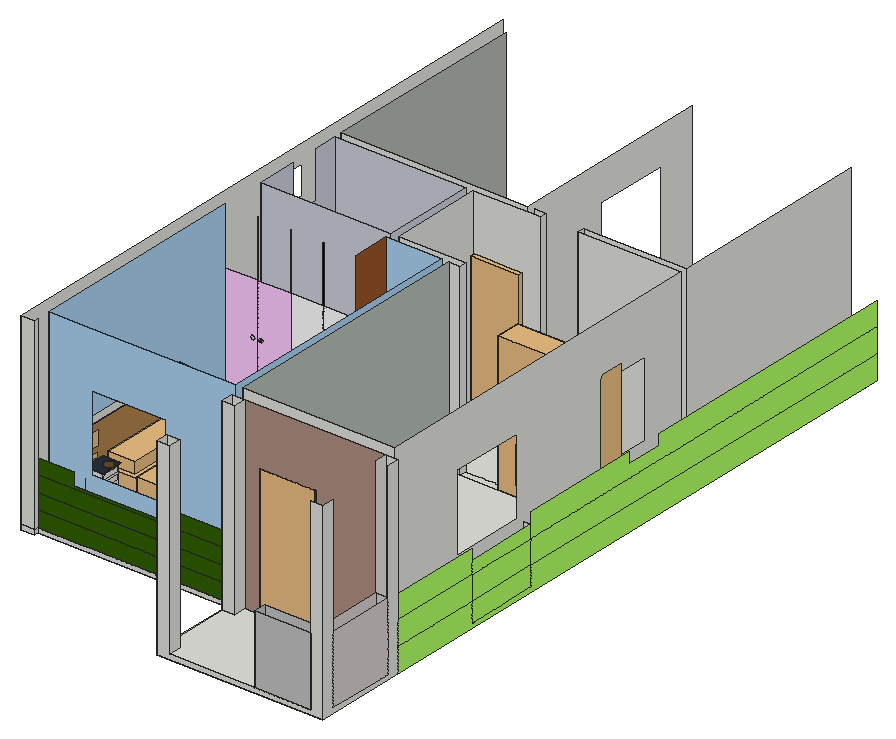
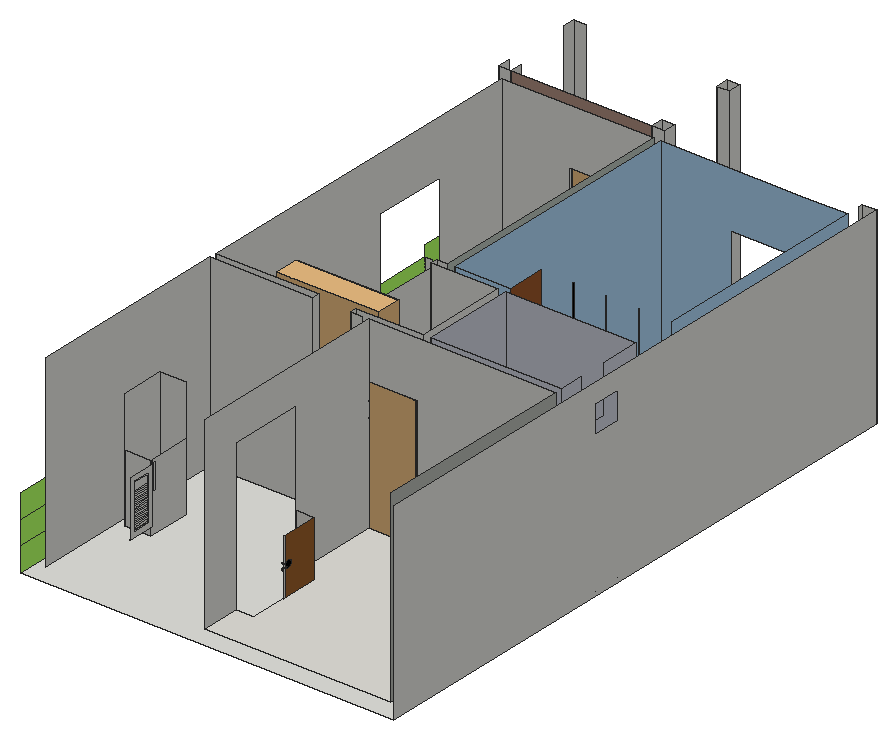
# SketchUp Ruby script. Lengths in inches.
U = 1.inch
M = Sketchup.active_model
def pt(a) = Geom::Point3d.new(a.map { |v| v * U })
def face(e, loops, mat)
  f = e.add_face(loops[0].map { |a| pt(a) })
  loops[1..].each { |l| e.add_face(l.map { |a| pt(a) }).erase! }
  f.material = f.back_material = mat if mat
  f
end
# faces: each face lists its corners as indices into pts; further lists are holes
def faces(e, pts, list, mat = nil) = list.each { |f| face(e, (f[0].is_a?(Array) ? f : [f]).map { |l| l.map { |i| pts[i] } }, mat) }
# xy, xz, yz: faces in a plane at the given z, y or x. An outline is a flat list of corners, or four numbers for a rectangle; further outlines are holes
def ring(l) = l.size == 4 ? [[l[0], l[1]], [l[2], l[1]], [l[2], l[3]], [l[0], l[3]]] : l.each_slice(2).to_a
def flat(e, list, mat, &to3) = list.each { |f| face(e, (f[0].is_a?(Array) ? f : [f]).map { |l| ring(l).map { |u, v| to3.(u, v) } }, mat) }
def xy(e, z, list, mat = nil) = flat(e, list, mat) { |x, y| [x, y, z] }
def xz(e, y, list, mat = nil) = flat(e, list, mat) { |x, z| [x, y, z] }
def yz(e, x, list, mat = nil) = flat(e, list, mat) { |y, z| [x, y, z] }
def lines(e, pts, list) = list.each { |a, b| e.add_line(pt(pts[a]), pt(pts[b])) }
# prism: a flat outline (further loops are holes) pulled along v
def prism(e, loops, v, mat = nil)
  f = face(e, loops, mat); d = Geom::Vector3d.new(v.map { |x| x * U })
  f.pushpull(f.normal.samedirection?(d) ? d.length : -d.length)
end
def box(e, o, s, mat = nil) = prism(e, [[o, [o[0] + s[0], o[1], o[2]], [o[0] + s[0], o[1] + s[1], o[2]], [o[0], o[1] + s[1], o[2]]]], [0, 0, s[2]], mat)
def at(x, y, z, deg = 0) = Geom::Transformation.translation(pt([x, y, z])) * Geom::Transformation.rotation(ORIGIN, Z_AXIS, deg.degrees)
def axes(o, x, y, z) = Geom::Transformation.new([*x, 0, *y, 0, *z, 0, *pt(o).to_a, 1])
def part(name) = M.definitions.add(name)
# library, detail: a bought-in or finely detailed component or shape, given as its bounding box
def library(name, o, s) = part(name).tap { |d| box(d.entities, o, s) }
def detail(e, o, s) = box(e.add_group.entities, o, s)
def put(e, d, t, mat = nil) = e.add_instance(d, t).tap { |i| i.material = mat if mat }
def group(e, t, mat = nil) = e.add_group.tap { |g| g.transformation = t; g.material = mat if mat }.entities
root = M.entities
M.materials.add("15___Default_0_2").color = [173, 175, 171]
M.materials.add("Color_4").color = [0, 0, 0]
M.materials.add("Material36").color = [96, 70, 37]
M.materials.add("Material__1").color = [125, 118, 110]
M.materials.add("PDM Brown VP_Books_03").color = [85, 37, 1]
M.materials.add("PDM Cover VP_Books_03").color = [103, 73, 44]
M.materials.add("PDM Pages VP_Books_03").color = [224, 224, 224]
M.materials.add("W143X910B75_NILAYA NEW MODERN 31846 ROLL B75").color = [180, 183, 177]
M.materials.add("W144X939F75_NILAYA EQUINOX FD25726 ROLL F75").color = [180, 190, 181]
M.materials.add("[Color F01]").color = [47, 96, 0]
M.materials.add("[Color F03]").color = [178, 255, 101]
M.materials.add("[Color K01]").color = [255, 204, 255]
M.materials.add("[Color M00]").color = [255, 255, 255]
M.materials.add("[Color M09]").color = [0, 0, 0]
M.materials.add("[Concrete Pavers Block Multi]").color = [124, 140, 145]
M.materials.add("[Fencing Metal Straight]").color = [194, 195, 196]
M.materials.add("[Fencing Railing Metal]").color = [216, 207, 208]
M.materials.add("[Herringbone]").color = [130, 130, 130]
M.materials.add("[Marble Carrara Floor Tile]").color = [204, 208, 219]
M.materials.add("[Marble Carrara Gold Floor Tile]").color = [225, 223, 217]
M.materials.add("[Pavers Modular Brick]").color = [175, 143, 129]
M.materials.add("[Resin Blue]").color = [171, 210, 241]
M.materials.add("[Wood Cherry Original]").color = [152, 86, 42]
M.materials.add("[Wood Floor Dark]").color = [153, 94, 42]
M.materials.add("elefante 02").color = [229, 229, 229]
M.materials.add("roblenatural1802").color = [180, 132, 79]
M.materials.add("wire_1").color = [39, 49, 60]
c1 = library("door2.dxf",[0,0,0],[35.42,7.875,78.74])
c2 = part("Chevet CHENONCEAU, Maisons du monde. Réf: 115.709 Prix: 129")
xy(c2.entities,0,[[1.3125,0.79,2.43,12.99],[15.54,0.79,16.57,12.99]])
xy(c2.entities,2.03,[[4.39,0.79,13.68,12.99]])
xy(c2.entities,3.26,[[2.51,0.79,15.51,12.52]])
xy(c2.entities,12.82,[[2.51,0.79,15.51,12.52]])
xy(c2.entities,14.17,[[2.51,0.67,15.42,0.79]])
xy(c2.entities,17.37,[[2.51,0.67,15.42,0.79]])
xy(c2.entities,18.73,[[2.53,0.72,15.34,0.79]])
xy(c2.entities,21.96,[[2.53,0.72,15.34,0.79]])
xy(c2.entities,22.57,[[1.3125,0.39,16.57,0.79],[16.57,0.39,16.89,12.99]])
xy(c2.entities,23.26,[[0,0,0.79,12.99],[0.79,0,17.11,0.39],[17.11,0,17.72,12.99]])
xy(c2.entities,23.62,[[0,0,17.72,12.99]],"wire_1")
xz(c2.entities,0,[[0,23.26,17.72,23.62]],"wire_1")
xz(c2.entities,0.39,[[1.3125,22.57,16.89,22.57,17.11,23.11,0.79,23.09],[0.79,23.09,17.11,23.11,17.11,23.26,0.79,23.26]])
xz(c2.entities,0.67,[[2.51,14.17,15.42,17.37]])
xz(c2.entities,0.72,[[2.53,18.73,15.34,21.96]])
xz(c2.entities,0.79,[[[1.3125,0,2.43,0,2.44,0.26,2.48,0.52,2.56,0.77,2.67,1.01,2.81,1.23,2.98,1.43,3.17,1.61,3.39,1.76,3.62,1.875,3.87,1.96,4.125,2.01,4.39,2.03,13.68,2.03,13.9375,2.01,14.1875,1.96,14.43,1.875,14.66,1.75,14.87,1.6,15.06,1.43,15.22,1.22,15.35,1,15.45,0.76,15.51,0.51,15.54,0.26,15.54,0,16.57,0,16.57,22.57,1.3125,22.57],[2.51,3.26,15.51,12.82],[2.53,18.73,15.34,21.96],[2.51,14.17,15.42,17.37]]])
xz(c2.entities,12.52,[[2.51,3.26,15.51,12.82]])
xz(c2.entities,12.99,[[1.3125,0,1.3125,22.57,0.79,23.09,0.79,23.26,0,23.26,0,23.62,17.72,23.62,17.72,23.26,17.11,23.26,17.11,23.11,16.89,22.57,16.57,22.57,16.57,0,15.54,0,15.54,0.26,15.51,0.51,15.45,0.76,15.35,1,15.22,1.22,15.06,1.43,14.87,1.6,14.66,1.75,14.43,1.875,14.1875,1.96,13.9375,2.01,13.68,2.03,4.39,2.03,4.125,2.01,3.87,1.96,3.62,1.875,3.39,1.76,3.17,1.61,2.98,1.43,2.81,1.23,2.67,1.01,2.56,0.77,2.48,0.52,2.44,0.26,2.43,0]])
yz(c2.entities,0,[[0,23.26,12.99,23.62]],"wire_1")
yz(c2.entities,0.79,[[0.39,23.09,12.99,23.26]])
yz(c2.entities,1.3125,[[0.79,0,12.99,22.57]])
yz(c2.entities,2.51,[[0.79,3.26,12.52,12.82],[0.67,14.17,0.79,17.37]])
yz(c2.entities,2.53,[[0.72,18.73,0.79,21.96]])
yz(c2.entities,15.34,[[0.72,18.73,0.79,21.96]])
yz(c2.entities,15.42,[[0.67,14.17,0.79,17.37]])
yz(c2.entities,15.51,[[0.79,3.26,12.52,12.82]])
yz(c2.entities,15.54,[[0.79,0,12.99,0.26]])
yz(c2.entities,16.57,[[0.79,0,12.99,22.57]])
yz(c2.entities,17.11,[[0.39,23.11,12.99,23.26]])
yz(c2.entities,17.72,[[0,23.26,12.99,23.62]],"wire_1")
p = [[2.43,12.99,0],[2.44,12.99,0.26],[2.44,0.79,0.26],[2.43,0.79,0],[2.48,12.99,0.52],[2.48,0.79,0.52],
  [15.51,12.99,0.51],[15.54,12.99,0.26],[15.54,0.79,0.26],[15.51,0.79,0.51],[2.56,12.99,0.77],[2.56,0.79,0.77],
  [15.45,12.99,0.76],[15.45,0.79,0.76],[2.67,12.99,1.01],[2.67,0.79,1.01],[15.35,12.99,1],[15.35,0.79,1],
  [2.81,12.99,1.23],[2.81,0.79,1.23],[15.22,12.99,1.22],[15.22,0.79,1.22],[2.98,12.99,1.43],[2.98,0.79,1.43],
  [15.06,12.99,1.43],[15.06,0.79,1.43],[3.17,12.99,1.61],[3.17,0.79,1.61],[14.87,12.99,1.6],[14.87,0.79,1.6],
  [3.39,12.99,1.76],[3.39,0.79,1.76],[14.66,12.99,1.75],[14.66,0.79,1.75],[3.62,12.99,1.875],[3.62,0.79,1.875],
  [14.43,12.99,1.875],[14.43,0.79,1.875],[3.87,12.99,1.96],[3.87,0.79,1.96],[14.1875,12.99,1.96],[14.1875,0.79,1.96],
  [4.125,12.99,2.01],[4.125,0.79,2.01],[4.39,12.99,2.03],[4.39,0.79,2.03],[13.68,12.99,2.03],[13.9375,12.99,2.01],
  [13.9375,0.79,2.01],[13.68,0.79,2.03],[1.3125,0.79,22.57],[1.3125,0.39,22.57],[0.79,0.39,23.09],[0.79,12.99,23.09],
  [1.3125,12.99,22.57],[17.11,12.99,23.11],[17.11,0.39,23.11],[16.89,0.39,22.57],[16.89,12.99,22.57]]
faces(c2.entities,p,[[0,1,2,3],[1,4,5,2],[6,7,8,9],[4,10,11,5],[12,6,9,13],[10,14,15,11],[16,12,13,17],[14,18,19,15],
  [20,16,17,21],[18,22,23,19],[24,20,21,25],[22,26,27,23],[28,24,25,29],[26,30,31,27],[32,28,29,33],[30,34,35,31],
  [36,32,33,37],[34,38,39,35],[40,36,37,41],[38,42,43,39],[42,44,45,43],[46,47,48,49],[47,40,41,48],[50,51,52,53,54],
  [55,56,57,58]])
c3 = library("Bega_2263.skp",[0,0,-4.33],[9.1,9.1,4.54])
c4 = library("ELK",[8.53,-0.73,3.43],[4.44,1.03,2.5])
c5 = part("VP_Books_03_Cover")
xy(c5.entities,-0.33,[[0,-1.3,11.69,7.49]],"PDM Brown VP_Books_03")
xy(c5.entities,-0.25,[[0,-1.22,11.69,7.49]],"PDM Brown VP_Books_03")
xy(c5.entities,1.04,[[0,-1.22,11.69,7.49]],"PDM Brown VP_Books_03")
xy(c5.entities,1.12,[[0,-1.3,11.69,7.49]],"PDM Cover VP_Books_03")
xz(c5.entities,-1.3,[[0,-0.33,11.69,1.12]],"PDM Cover VP_Books_03")
xz(c5.entities,-1.22,[[0,-0.25,11.69,1.04]],"PDM Brown VP_Books_03")
xz(c5.entities,7.49,[[0,-0.33,11.69,-0.25],[0,1.04,11.69,1.12]],"PDM Brown VP_Books_03")
yz(c5.entities,0,[[-1.3,-0.33,-1.3,1.12,7.49,1.12,7.49,1.04,-1.22,1.04,-1.22,-0.25,7.49,-0.25,7.49,-0.33]],"PDM Cover VP_Books_03")
yz(c5.entities,11.69,[[-1.3,-0.33,7.49,-0.33,7.49,-0.25,-1.22,-0.25,-1.22,1.04,7.49,1.04,7.49,1.12,-1.3,1.12]],"PDM Cover VP_Books_03")
c6 = part("VP_Books_03_Pages")
box(c6.entities,[0,-1.3,-0.33],[11.46,8.59,1.29],"PDM Pages VP_Books_03")
c7 = part("VP_Books_03.skp")
put(c7.entities,c5,axes([0,1.57,0.39],[1.21,0,0],[0,1.21,0],[0,0,1.21]))
put(c7.entities,c6,axes([0.14,1.67,0.49],[1.21,0,0],[0,1.21,0],[0,0,1.21]))
c8 = library("Group\#23",[-408.7,46.15,517.94],[1547.31,468.28,362.21])
c9 = library("Group\#21",[-519.15,-1391.32,251.35],[1756.04,1892.7,383.55])
c10 = library("Group\#20",[-576.09,-1463.59,4.12],[1840.9,2045.19,319.09])
c11 = library("Group\#19",[-609.9,-1576.45,97.75],[1838.77,1457.89,642.22])
c12 = library("Group\#12",[-612.85,-1140.67,180.96],[1888,514.01,543.34])
c13 = library("Group\#15",[-455.57,-1315.72,309.1],[1631.9,1798.78,127.41])
c14 = part("BED-0235")
put(c14.entities,c8,at(0,0,0),"wire_1")
g1 = group(c14.entities,at(0,0,0),"wire_1")
p = [[710.91,736.79,563.57],[711.15,735.84,567.82],[713.76,733.43,565.7],[231.46,704.77,566.08],[225.3,708.01,564.82],[226.88,706.82,568.1875],
  [225.36,706.93,576.125]]
faces(g1,p,[[0,1,2],[3,4,5],[6,3,5]],"15___Default_0_2")
put(c14.entities,c9,at(0,0,0),"wire_1")
put(c14.entities,c10,at(0,0,0),"wire_1")
put(c14.entities,c11,at(0,0,0),"wire_1")
put(c14.entities,c12,at(0,0,0),"Material__1")
put(c14.entities,c13,at(0,0,0),"wire_1")
c15 = library("Alarm_clock_retro.skp",[-0.85,-1.11,-0.01],[5.38,3.78,6.48])
c16 = library("skp790C",[-18.38,-3.42,-42.32],[36.76,6.84,84.64])
c17 = library("Group\#809",[-2.43,-5.1,0],[16.85,20.23,24.37])
c18 = library("Group\#792",[-0.01,-0.01,0],[14.14,13.75,2.62])
c19 = library("Group_56\#1",[41.72,11.43,21.26],[15.24,13.44,5.45])
c20 = library("Group\#824",[0,0,0],[2.46,6.04,7.11])
c21 = library("Group\#50",[0,0,0],[107.72,88.39,15.75])
c22 = library("vase3mm",[-1.8,-1.8,0],[3.6,3.6,4.77])
c23 = library("Group\#207",[0,-0.71,-0.55],[4.57,9.54,14.74])
c24 = library("Group\#4",[0,0,0],[80.15,172,15.875])
xy(root,35.43,[[133.5,0,240,60],[0,57,0,444,240,444,240,60,9,60,9,57]])
xy(root,38.43,[[141.5,0,196,0,196,8,232,8,232,60,141.5,60,141.5,52,133.5,52,133.5,8,141.5,8],[196,0,232,8],[84.01,60,133.5,60,133.5,68,141.5,68,141.5,60,151.5,60,151.5,69,133.5,69,133.5,234,140.7,234,140.7,238.5,129,238.5,129,69,84.01,69],[133.5,60,141.5,68],[151.5,60,187.5,69],
  [232,60,240,68],[133.5,69,231,234],[231,118.97,240,166.97],[99,234,129,234,129,238.5,231,238.5,231,298.5,129,298.5,129,303,99,303,99,298.5,97.5,298.5,97.5,286.5,93,286.5,93,250.5,97.5,250.5,97.5,238.5,99,238.5],[140.7,234,164.7,238.5],
  [164.7,234,231,238.5],[140.7,298.5,164.7,303],[208.97,349.92,225.68,378.03]])
xy(root,38.43,[[9,69,129,69,129,234,93,234,93,210,9,210]],"[Concrete Pavers Block Multi]")
xy(root,38.43,[[232,8,240,52]],"[Fencing Railing Metal]")
xy(root,38.43,[[9,238.5,93,298.5]],"[Herringbone]")
xy(root,38.43,[[9,303,129,303,129,361.98,117,361.98,117,409.98,129,409.98,129,435,9,435]],"[Marble Carrara Gold Floor Tile]")
xy(root,38.87,[[9,90.07,14.125,106.6],[9,106.6,14.125,174.1]])
xy(root,43.89,[[208.39,378.03,208.97,394.875]])
xy(root,63.72,[[13.76,165.71,14.125,165.83]],"roblenatural1802")
xz(root,0,[[133.5,35.43,240,35.43,240,158.43,232,158.43,232,38.43,141.5,38.43,141.5,158.43,133.5,158.43]])
xz(root,0,[[196,38.43,232,82.43]],"[Fencing Metal Straight]")
xz(root,8,[[133.5,38.43,141.5,158.43]])
xz(root,8,[[196,38.43,232,82.43]],"[Fencing Metal Straight]")
xz(root,8,[[232,38.43,240,82.43]],"[Fencing Railing Metal]")
xz(root,52,[[133.5,38.43,141.5,158.43]])
xz(root,52,[[232,38.43,240,82.43]],"[Fencing Railing Metal]")
xz(root,57,[[0,35.43,9,38.43],[0,38.43,9,158.43]])
xz(root,60,[[9,35.43,133.5,38.43],[133.5,35.43,240,38.43],[133.5,38.43,141.5,158.43],[232,38.43,240,158.43]])
xz(root,60,[[9,38.43,133.5,48.43],[9,48.43,133.5,58.43],[9,58.43,133.5,68.43],[9,68.43,133.5,68.43,133.5,78.43,88.01,78.43,88.01,70.43,32.01,70.43,32.01,78.43,9,78.43]],"[Color F01]")
xz(root,60,[[141.5,38.43,151.5,38.43,151.5,122.43,187.5,122.43,187.5,38.43,232,38.43,232,158.43,141.5,158.43]],"[Pavers Modular Brick]")
xz(root,69,[[36.01,37.43,84.01,38.43],[133.5,38.43,133.5,158.43,231,158.43,231,38.43,187.5,38.43,187.5,122.43,151.5,122.43,151.5,38.43]])
xz(root,69,[[9,38.43,9,158.43,36.01,158.43,36.01,74.43,84.01,74.43,84.01,122.43,36.01,122.43,36.01,158.43,129,158.43,129,38.43]],"[Resin Blue]")
xz(root,90.07,[[9,38.87,14.125,83.36]],"wire_1")
xz(root,118.97,[[235.5,38.43,240,74.43]])
xz(root,165.28,[[13.76,64.2,14.125,64.36]],"roblenatural1802")
xz(root,166.97,[[235.5,38.43,240,74.43]])
xz(root,174.1,[[9,38.87,14.125,83.36]],"wire_1")
xz(root,210,[[[9,38.43,30,122.13],[25.97,86.42,25.04,88.02,25.96,89.61,27.8,89.62,28.72,88.03,27.81,86.43]],[[30.3,38.43,51,122.13],[33.0625,86.43,31.24,86.45,30.35,88.05,31.28,89.61,33.1,89.59,33.99,88]]],"[Color K01]")
xz(root,210,[[[51.3,38.43,72,122.13],[69.76,86.43,67.9,86.45,66.98,88.07,67.93,89.67,69.79,89.65,70.7,88.03]],[[72.3,38.43,93,122.13],[74.6,86.41,73.64,88.03,74.5625,89.67,76.45,89.69,77.41,88.07,76.49,86.43]]],"[Color M00]")
xz(root,210,[[30,38.43,30.3,158.43],[51,38.43,51.3,158.43],[72,38.43,72.3,158.43]],"[Color M09]")
xz(root,234,[[133.5,38.43,140.7,158.43]])
xz(root,234,[[93,38.43,99,38.43,99,122.43,129,122.43,129,158.43,93,158.43]],"[Resin Blue]")
xz(root,238.5,[[97.5,38.43,97.5,158.43,140.7,158.43,140.7,38.43,129,38.43,129,122.43,99,122.43,99,38.43]])
xz(root,238.5,[[9,38.43,93,158.43]],"[Marble Carrara Floor Tile]")
xz(root,250.5,[[93,38.43,97.5,122.43]])
xz(root,286.5,[[93,38.43,97.5,122.43]])
xz(root,298.5,[[97.5,38.43,99,38.43,99,122.43,129,122.43,129,38.43,140.7,38.43,140.7,158.43,97.5,158.43],[164.7,38.43,231,158.43]])
xz(root,298.5,[[9,38.43,93,158.43]],"[Marble Carrara Floor Tile]")
xz(root,303,[[9,38.43,9,158.43,129,158.43,129,122.43,99,122.43,99,38.43],[133.5,38.43,140.7,158.43],[164.7,38.43,231,158.43]])
xz(root,349.92,[[208.97,38.43,225.68,114.79]])
xz(root,361.98,[[117,38.43,129,74.43]],"[Marble Carrara Gold Floor Tile]")
xz(root,378.03,[[208.97,38.43,225.68,82.07],[208.39,43.89,208.97,82.07]])
yz(root,0,[[[57,35.43,444,158.43],[264.68,128.44,282.68,146.43]]])
yz(root,9,[[57,35.43,60,38.43],[57,38.43,60,158.43],[90.07,38.87,174.1,83.36]])
yz(root,9,[[303,38.43,435,158.43]],"W143X910B75_NILAYA NEW MODERN 31846 ROLL B75")
yz(root,9,[[238.5,38.43,298.5,38.43,298.5,158.43,282.68,158.43,282.68,128.43,264.68,128.43,264.68,158.43,238.5,158.43]],"[Marble Carrara Floor Tile]")
yz(root,9,[[[69,38.43,210,158.43],[90.07,38.87,174.1,83.36]]],"[Resin Blue]")
yz(root,13.39,[[97.33,63.72,97.46,63.74,97.57,63.8,97.67,63.89,97.75,64.02,97.8,64.16,97.82,64.31,97.8,64.47,97.75,64.61,97.67,64.74,97.57,64.83,97.46,64.89,97.33,64.91,97.21,64.89,97.09,64.83,96.99,64.74,96.91,64.61,96.86,64.47,96.85,64.31,96.86,64.16,96.91,64.02,96.99,63.89,97.09,63.8,97.21,63.74]],"roblenatural1802")
yz(root,13.76,[[165.71,63.72,165.83,63.72,165.95,63.77,166.06,63.85,166.14,63.96,166.2,64.1,166.23,64.25,166.22,64.4,166.1875,64.55,166.12,64.68,166.03,64.78,165.92,64.85,165.8,64.89,165.67,64.88,165.55,64.84,165.45,64.76,165.36,64.64,165.31,64.51,165.28,64.36,165.28,64.2,165.32,64.06,165.38,63.93,165.48,63.82,165.59,63.75]],"roblenatural1802")
yz(root,14.125,[[[90.68,39.62,173.49,82.61],[97.33,63.72,97.21,63.74,97.09,63.8,96.99,63.89,96.91,64.02,96.86,64.16,96.85,64.31,96.86,64.47,96.91,64.61,96.99,64.74,97.09,64.83,97.21,64.89,97.33,64.91,97.46,64.89,97.57,64.83,97.67,64.74,97.75,64.61,97.8,64.47,97.82,64.31,97.8,64.16,97.75,64.02,97.67,63.89,97.57,63.8,97.46,63.74],[165.71,63.72,165.59,63.75,165.48,63.82,165.38,63.93,165.32,64.06,165.28,64.2,165.28,64.36,165.31,64.51,165.36,64.64,165.45,64.76,165.55,64.84,165.67,64.88,165.8,64.89,165.92,64.85,166.03,64.78,166.12,64.68,166.1875,64.55,166.22,64.4,166.23,64.25,166.2,64.1,166.14,63.96,166.06,63.85,165.95,63.77,165.83,63.72]]],"roblenatural1802")
yz(root,14.125,[[[90.07,38.87,174.1,83.36],[90.68,39.62,173.49,82.61]]],"wire_1")
yz(root,36.01,[[64.09,37.43,69,38.43]])
yz(root,93,[[238.5,38.43,238.5,158.43,298.5,158.43,298.5,38.43,286.5,38.43,286.5,122.43,250.5,122.43,250.5,38.43]],"[Marble Carrara Floor Tile]")
yz(root,93,[[210,38.43,234,158.43]],"[Wood Cherry Original]")
yz(root,97.5,[[238.5,38.43,250.5,38.43,250.5,122.43,286.5,122.43,286.5,38.43,298.5,38.43,298.5,158.43,238.5,158.43]])
yz(root,99,[[234,38.43,238.5,122.43],[298.5,38.43,303,122.43]])
yz(root,116.5,[[383.21,55.43,382.6875,55.47,382.2,55.64,381.76,55.9375,381.42,56.33,381.2,56.8,381.1,57.32,381.14,57.84,381.31,58.33,381.6,58.76,382,59.1,382.47,59.33,382.98,59.43,383.5,59.39,384,59.21,384.43,58.92,384.77,58.53,385,58.05,385.09,57.54,385.05,57.02,384.88,56.53,384.59,56.1,384.19,55.76,383.72,55.53]],"[Color M09]")
yz(root,117,[[385.68,38.43,385.98,74.43]],"[Marble Carrara Gold Floor Tile]")
yz(root,117,[[[361.98,38.43,385.68,74.43],[383.21,55.43,383.72,55.53,384.19,55.76,384.59,56.1,384.88,56.53,385.05,57.02,385.09,57.54,385,58.05,384.77,58.53,384.43,58.92,384,59.21,383.5,59.39,382.98,59.43,382.47,59.33,382,59.1,381.6,58.76,381.31,58.33,381.14,57.84,381.1,57.32,381.2,56.8,381.42,56.33,381.76,55.9375,382.2,55.64,382.6875,55.47]]],"[Wood Floor Dark]")
yz(root,129,[[234,38.43,238.5,122.43],[298.5,38.43,303,122.43],[303,38.43,303,158.43,435,158.43,435,38.43,409.98,38.43,409.98,134.43,361.98,134.43,361.98,38.43]])
yz(root,129,[[69,38.43,234,158.43]],"[Resin Blue]")
yz(root,133.5,[[0,35.43,0,158.43,8,158.43,8,38.43,52,38.43,52,158.43,60,158.43,60,35.43]])
yz(root,133.5,[[69,38.43,234,158.43]],"W144X939F75_NILAYA EQUINOX FD25726 ROLL F75")
yz(root,140.7,[[234,38.43,238.5,158.43],[298.5,38.43,303,158.43]])
yz(root,141.5,[[0,38.43,8,158.43],[52,38.43,60,158.43]])
yz(root,151.5,[[60,38.43,69,122.43]])
yz(root,164.7,[[298.5,38.43,303,158.43]])
yz(root,187.5,[[60,38.43,69,122.43]])
yz(root,196,[[0,38.43,8,82.43]],"[Fencing Metal Straight]")
yz(root,208.39,[[[378.03,43.89,394.875,79.89],[380.4375,47.16,392.46,76.61]],[[380.4375,47.16,392.46,76.61],[380.84,47.7,392.0625,76.07]],[380.84,47.7,381.11,76.07],[381.11,47.7,392.0625,48.79],[381.11,48.79,392.0625,49.89],
  [381.11,49.89,392.0625,50.98],[381.11,50.98,392.0625,52.07],[381.11,52.07,392.0625,53.16],[381.11,53.16,392.0625,54.25],[381.11,54.25,392.0625,55.34],
  [381.11,55.34,392.0625,56.43],[381.11,56.43,392.0625,57.52],[381.11,57.52,392.0625,58.61],[381.11,58.61,392.0625,59.7],[381.11,59.7,392.0625,60.79],
  [381.11,60.79,392.0625,61.89],[381.11,61.89,392.0625,62.98],[381.11,62.98,392.0625,64.07],[381.11,64.07,392.0625,65.16],[381.11,65.16,392.0625,66.25],
  [381.11,66.25,392.0625,67.34],[381.11,67.34,392.0625,68.43],[381.11,68.43,392.0625,69.52],[381.11,69.52,392.0625,70.61]])
yz(root,208.97,[[[349.92,38.43,378.03,82.07],[374.37,63.28,376.05,80.19]],[374.37,63.28,376.05,80.19]])
yz(root,225.68,[[349.92,38.43,378.03,114.79]])
yz(root,231,[[[69,38.43,298.5,158.43],[118.97,74.43,166.97,123.43],[245.63,74.43,269.63,122.43]],[303,38.43,435,158.43]])
yz(root,232,[[0,38.43,8,82.43],[52,38.43,60,158.43]])
yz(root,232,[[8,38.43,52,82.43]],"[Fencing Railing Metal]")
yz(root,240,[[0,35.43,60,35.43,60,158.43,52,158.43,52,38.43,8,38.43,8,158.43,0,158.43]])
yz(root,240,[[60,35.43,444,35.43,444,50.81,166.97,50.81,166.97,38.43,118.97,38.43,118.97,50.81,60,50.81],[118.97,38.43,166.97,50.81],[60,50.81,118.97,66.18],[118.97,50.81,166.97,66.18],[166.97,50.81,444,66.18],
  [60,66.18,118.97,81.56],[118.97,66.18,166.97,74.43],[166.97,66.18,444,66.18,444,81.56,269.63,81.56,269.63,74.43,245.63,74.43,245.63,81.56,166.97,81.56]],"[Color F03]")
yz(root,240,[[8,38.43,52,82.43]],"[Fencing Railing Metal]")
p = [[117,383.21,55.43],[117,382.6875,55.47],[116.5,382.6875,55.47],[116.5,383.21,55.43],[117,383.72,55.53],[116.5,383.72,55.53],
  [117,382.2,55.64],[116.5,382.2,55.64],[117,384.19,55.76],[116.5,384.19,55.76],[117,381.76,55.9375],[116.5,381.76,55.9375],
  [117,388.06,55.74],[117,387.58,55.95],[116.5,387.58,55.95],[116.5,388.06,55.74],[117,384.59,56.1],[116.5,384.59,56.1],
  [117,381.42,56.33],[116.5,381.42,56.33],[117,387.17,56.26],[116.5,387.17,56.26],[117,384.88,56.53],[116.5,384.88,56.53],
  [117,381.2,56.8],[116.5,381.2,56.8],[117,386.85,56.68],[116.5,386.85,56.68],[117,385.05,57.02],[116.5,385.05,57.02],
  [117,386.65,57.16],[116.5,386.65,57.16],[117,381.1,57.32],[116.5,381.1,57.32],[117,385.09,57.54],[116.5,385.09,57.54],
  [117,386.59,57.68],[116.5,386.59,57.68],[117,381.14,57.84],[116.5,381.14,57.84],[117,385,58.05],[116.5,385,58.05],
  [117,386.66,58.2],[116.5,386.66,58.2],[117,381.31,58.33],[116.5,381.31,58.33],[117,384.77,58.53],[116.5,384.77,58.53],
  [117,386.86,58.68],[116.5,386.86,58.68],[117,381.6,58.76],[116.5,381.6,58.76],[117,384.43,58.92],[116.5,384.43,58.92],
  [117,387.18,59.09],[116.5,387.18,59.09],[117,382,59.1],[116.5,382,59.1],[117,384,59.21],[116.5,384,59.21],
  [117,382.47,59.33],[116.5,382.47,59.33],[117,387.59,59.41],[116.5,387.59,59.41],[117,383.5,59.39],[116.5,383.5,59.39],
  [117,382.98,59.43],[116.5,382.98,59.43],[117,388.07,59.61],[116.5,388.07,59.61],[14.125,97.09,63.8],[14.125,97.21,63.74],
  [13.39,97.21,63.74],[13.39,97.09,63.8],[14.125,97.33,63.72],[13.39,97.33,63.72],[14.125,97.46,63.74],[13.39,97.46,63.74],
  [14.125,97.57,63.8],[13.39,97.57,63.8],[14.125,165.59,63.75],[14.125,165.71,63.72],[13.76,165.71,63.72],[13.76,165.59,63.75],
  [14.125,165.83,63.72],[14.125,165.95,63.77],[13.76,165.95,63.77],[13.76,165.83,63.72],[14.125,96.99,63.89],[13.39,96.99,63.89],
  [14.125,97.67,63.89],[13.39,97.67,63.89],[14.125,165.38,63.93],[14.125,165.48,63.82],[13.76,165.48,63.82],[13.76,165.38,63.93],
  [14.125,166.06,63.85],[13.76,166.06,63.85],[14.125,166.14,63.96],[13.76,166.14,63.96],[14.125,96.91,64.02],[13.39,96.91,64.02],
  [14.125,97.75,64.02],[13.39,97.75,64.02],[14.125,165.32,64.06],[13.76,165.32,64.06],[14.125,96.86,64.16],[13.39,96.86,64.16],
  [14.125,97.8,64.16],[13.39,97.8,64.16],[14.125,166.2,64.1],[13.76,166.2,64.1],[14.125,165.28,64.2],[13.76,165.28,64.2],
  [14.125,166.23,64.25],[13.76,166.23,64.25],[14.125,96.85,64.31],[13.39,96.85,64.31],[14.125,97.82,64.31],[13.39,97.82,64.31],
  [14.125,166.22,64.4],[13.76,166.22,64.4],[14.125,96.86,64.47],[13.39,96.86,64.47],[14.125,97.8,64.47],[13.39,97.8,64.47],
  [14.125,165.31,64.51],[14.125,165.28,64.36],[13.76,165.28,64.36],[13.76,165.31,64.51],[14.125,166.1875,64.55],[13.76,166.1875,64.55],
  [14.125,96.91,64.61],[13.39,96.91,64.61],[14.125,97.75,64.61],[13.39,97.75,64.61],[14.125,165.36,64.64],[13.76,165.36,64.64],
  [14.125,166.12,64.68],[13.76,166.12,64.68],[14.125,96.99,64.74],[13.39,96.99,64.74],[14.125,97.67,64.74],[13.39,97.67,64.74],
  [14.125,165.45,64.76],[13.76,165.45,64.76],[14.125,97.09,64.83],[13.39,97.09,64.83],[14.125,97.57,64.83],[13.39,97.57,64.83],
  [14.125,166.03,64.78],[13.76,166.03,64.78],[14.125,97.21,64.89],[13.39,97.21,64.89],[14.125,97.46,64.89],[13.39,97.46,64.89],
  [14.125,165.55,64.84],[13.76,165.55,64.84],[14.125,165.67,64.88],[13.76,165.67,64.88],[14.125,165.92,64.85],[13.76,165.92,64.85],
  [14.125,97.33,64.91],[13.39,97.33,64.91],[14.125,165.8,64.89],[13.76,165.8,64.89],[36.01,60,38.43],[36.01,64.09,38.43],
  [84.01,60,37.43],[84.01,69,37.43],[36.01,60,37.43],[36.01,64.09,37.43],[36.01,64.09,74.43],[9,264.68,38.43],
  [0,264.68,38.43],[0,282.68,38.43],[9,282.68,38.43],[14.125,95.73,40.05],[14.125,106.6,40.05],[84.38,157.78,38.87],
  [14.125,157.78,38.87],[14.125,157.78,40.05],[14.125,173.14,40.05]]
faces(root,p,[[0,1,2,3],[4,0,3,5],[1,6,7,2],[8,4,5,9],[6,10,11,7],[12,13,14,15],[16,8,9,17],[10,18,19,11],
  [13,20,21,14],[22,16,17,23],[18,24,25,19],[20,26,27,21],[28,22,23,29],[26,30,31,27],[24,32,33,25],[34,28,29,35],
  [30,36,37,31],[32,38,39,33],[40,34,35,41],[36,42,43,37],[38,44,45,39],[46,40,41,47],[42,48,49,43],[44,50,51,45],
  [52,46,47,53],[48,54,55,49],[50,56,57,51],[58,52,53,59],[56,60,61,57],[54,62,63,55],[64,58,59,65],[60,66,67,61],
  [66,64,65,67],[62,68,69,63]],"[Color M09]")
faces(root,p,[[70,71,72,73],[71,74,75,72],[74,76,77,75],[76,78,79,77],[80,81,82,83],[84,85,86,87],[88,70,73,89],[78,90,91,79],
  [92,93,94,95],[93,80,83,94],[85,96,97,86],[96,98,99,97],[100,88,89,101],[90,102,103,91],[104,92,95,105],[106,100,101,107],
  [102,108,109,103],[98,110,111,99],[112,104,105,113],[110,114,115,111],[116,106,107,117],[108,118,119,109],[114,120,121,115],[122,116,117,123],
  [118,124,125,119],[126,127,128,129],[120,130,131,121],[132,122,123,133],[124,134,135,125],[136,126,129,137],[130,138,139,131],[140,132,133,141],
  [134,142,143,135],[144,136,137,145],[146,140,141,147],[142,148,149,143],[138,150,151,139],[152,146,147,153],[148,154,155,149],[156,144,145,157],
  [158,156,157,159],[150,160,161,151],[162,152,153,163],[154,162,163,155],[164,158,159,165],[160,164,165,161]],"roblenatural1802")
lines(root,p,[[166,167],[168,169],[170,171],[172,167],[173,174],[175,176],[177,178],[179,180],[178,181],[181,182]])
put(root,c1,axes([151.5,60,38.43],[1,0,0],[0,1,0],[0,0,1.0668]))
put(root,c2,axes([26.11,90.38,38.5],[0,0.8125,0],[-0.9295,0,0],[0,0,1]))
put(root,c3,axes([14.125,94.18,69.09],[0,0.8125,0],[0,0,1],[0.9295,0,0]))
put(root,c4,axes([14.04,89.42,59.65],[0,0.8125,0],[-0.9295,0,0],[0,0,1]))
put(root,c7,axes([27.4375,98.11,62.12],[-0.36793,0.37924,0],[-0.38179,-0.28302,0],[0,0,0.17]))
put(root,c14,axes([33.73,121.28,38.46],[0,0.03085,0],[-0.03727,0,0],[0,0,0.02765]))
put(root,c15,axes([20.71,163.99,62.12],[0,0.8125,0],[-0.9295,0,0],[0,0,1]))
put(root,c2,axes([26.11,158.84,38.5],[0,0.8125,0],[-0.9295,0,0],[0,0,1]))
put(root,c3,axes([14.125,162.63,69.09],[0,0.8125,0],[0,0,1],[0.9295,0,0]))
put(root,c4,axes([14.04,157.88,59.65],[0,0.8125,0],[-0.9295,0,0],[0,0,1]))
put(root,c16,axes([113.65,235.125,80.43],[-0.84,0,0],[0,1,0],[0,0,0.99237]))
put(root,c17,axes([181.3125,234.49,48.59],[0.57884,0,0],[0,0.9173,0],[0,0,0.94044]))
put(root,c18,axes([190.375,240.67,48.59],[0.62365,1.06298,0],[0.64355,-1.04556,0],[0,0,1.49184]))
put(root,c19,axes([185.89,227.83,30.65],[0.49617,0,0],[0,0.75935,0],[0,0,0.84372]),"Color_4")
put(root,c20,axes([221.16,243.53,48.59],[0,-1.188,0],[0.71322,0,0],[0,0,1.2386]),"Material36")
put(root,c21,axes([164.7,250.2,38.43],[0.6155,0,0],[0,0,1],[0,-1,0]))
put(root,c22,axes([168.52,243.75,64.75],[0,2.2743,0],[-1.39984,0,0],[0,0,1.56927]))
put(root,c23,axes([174.1,240.54,49.3],[0.65145,0,0],[0,1.0584,0],[0,0,1.0584]),"elefante 02")
put(root,c24,axes([89.4,250.5,38.43],[0,0.44915,0],[0,0,0.48837],[0.51,0,0]))
put(root,c16,axes([113.57,299.62,80.43],[-0.84,0,0],[0,1,0],[0,0,0.99237]))
